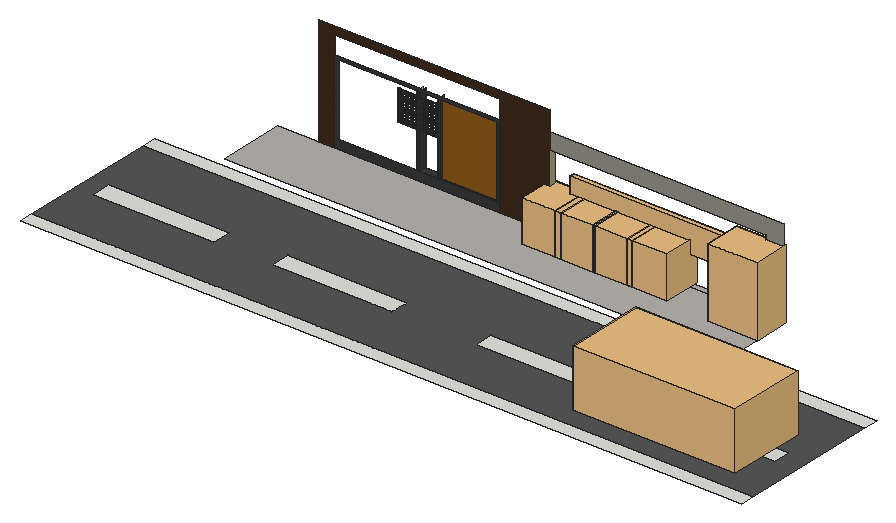
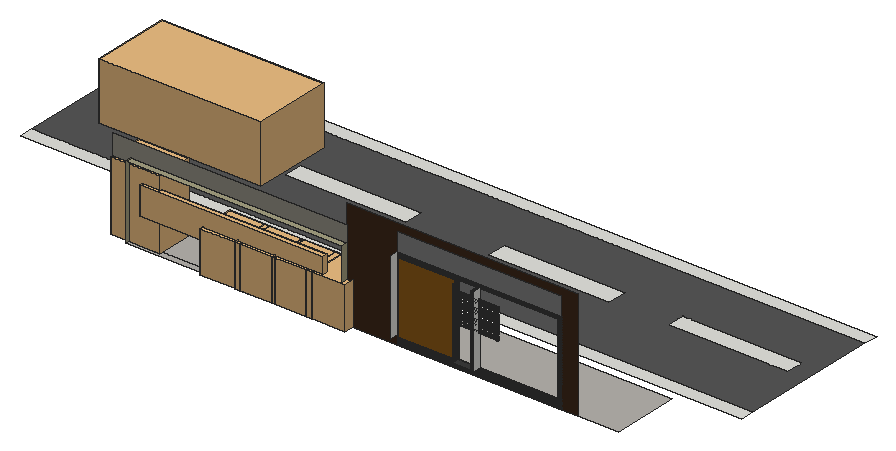
# SketchUp Ruby script. Lengths in inches.
U = 1.inch
M = Sketchup.active_model
def pt(a) = Geom::Point3d.new(a.map { |v| v * U })
def face(e, loops, mat)
  f = e.add_face(loops[0].map { |a| pt(a) })
  loops[1..].each { |l| e.add_face(l.map { |a| pt(a) }).erase! }
  f.material = f.back_material = mat if mat
  f
end
# faces: each face lists its corners as indices into pts; further lists are holes
def faces(e, pts, list, mat = nil) = list.each { |f| face(e, (f[0].is_a?(Array) ? f : [f]).map { |l| l.map { |i| pts[i] } }, mat) }
# xy, xz, yz: faces in a plane at the given z, y or x. An outline is a flat list of corners, or four numbers for a rectangle; further outlines are holes
def ring(l) = l.size == 4 ? [[l[0], l[1]], [l[2], l[1]], [l[2], l[3]], [l[0], l[3]]] : l.each_slice(2).to_a
def flat(e, list, mat, &to3) = list.each { |f| face(e, (f[0].is_a?(Array) ? f : [f]).map { |l| ring(l).map { |u, v| to3.(u, v) } }, mat) }
def xy(e, z, list, mat = nil) = flat(e, list, mat) { |x, y| [x, y, z] }
def xz(e, y, list, mat = nil) = flat(e, list, mat) { |x, z| [x, y, z] }
def yz(e, x, list, mat = nil) = flat(e, list, mat) { |y, z| [x, y, z] }
def lines(e, pts, list) = list.each { |a, b| e.add_line(pt(pts[a]), pt(pts[b])) }
# prism: a flat outline (further loops are holes) pulled along v
def prism(e, loops, v, mat = nil)
  f = face(e, loops, mat); d = Geom::Vector3d.new(v.map { |x| x * U })
  f.pushpull(f.normal.samedirection?(d) ? d.length : -d.length)
end
def box(e, o, s, mat = nil) = prism(e, [[o, [o[0] + s[0], o[1], o[2]], [o[0] + s[0], o[1] + s[1], o[2]], [o[0], o[1] + s[1], o[2]]]], [0, 0, s[2]], mat)
def at(x, y, z, deg = 0) = Geom::Transformation.translation(pt([x, y, z])) * Geom::Transformation.rotation(ORIGIN, Z_AXIS, deg.degrees)
def axes(o, x, y, z) = Geom::Transformation.new([*x, 0, *y, 0, *z, 0, *pt(o).to_a, 1])
def part(name) = M.definitions.add(name)
# library, detail: a bought-in or finely detailed component or shape, given as its bounding box
def library(name, o, s) = part(name).tap { |d| box(d.entities, o, s) }
def detail(e, o, s) = box(e.add_group.entities, o, s)
def put(e, d, t, mat = nil) = e.add_instance(d, t).tap { |i| i.material = mat if mat }
def group(e, t, mat = nil) = e.add_group.tap { |g| g.transformation = t; g.material = mat if mat }.entities
root = M.entities
M.materials.add("[Blinds Weave]").color = [141, 91, 25]
M.materials.add("[Color M06]").color = [86, 86, 86]
M.materials.add("[Color M07]").color = [58, 58, 58]
M.materials.add("[Formica Graystone]1").color = [149, 146, 135]
M.materials.add("[Formica Speckled Grey]").color = [94, 105, 111]
M.materials.add("[Sandstone]").color = [63, 43, 28]
M.materials.add("[Stone Coursed Rough]").color = [165, 160, 130]
M.materials.add("[Tile Travertine 2 inch]").color = [181, 178, 172]
c1 = library("Small+Bush+Planter",[-31.86,3.96,0],[62.63,58.8,106.375])
c2 = library("MVSR Maanus",[1.41,0,0],[199.01,20.125,12])
c3 = library("chau cay",[-24.34,-109.24,0],[56.46,62.58,79.69])
c4 = library("2015 Porsche Macan",[0.14,0.6,0.32],[90.05,184.43,65.58])
xy(root,0,[[0,0,824.125,15.99],[21.05,78.34,158.24,100.09],[225.11,78.34,362.3,100.09],[458.05,78.34,595.24,100.09],[662.36,78.34,799.55,100.09],
  [0,176.43,824.125,192.625]])
xy(root,0,[[[0,15.99,824.125,176.43],[21.05,78.34,158.24,100.09],[225.11,78.34,362.3,100.09],[458.05,78.34,595.24,100.09],[662.36,78.34,799.55,100.09]]],"[Color M06]")
xy(root,0,[[71.32,202.61,649.65,279.21],[381.67,279.21,628.99,285.9]],"[Tile Travertine 2 inch]")
xy(root,10.08,[[229.25,279.21,232.82,288.34]])
xy(root,10.08,[[232.82,279.21,253.76,288.34],[256.89,279.21,321.11,281.7]],"[Color M07]")
xy(root,83.9375,[[381.67,279.21,628.99,285.9]],"[Stone Coursed Rough]")
xz(root,279.21,[[136.3,0,324.42,10.08],[136.3,10.08,140.74,10.08,140.74,91.34,321.11,91.34,321.11,10.08,324.42,10.08,324.42,94.91,136.3,94.91],[229.25,10.08,232.82,91.34],[253.76,10.08,256.89,91.34]],"[Color M07]")
xz(root,279.21,[[628.99,0,649.65,0,649.65,103.14,381.67,103.14,381.67,83.9375,628.99,83.9375]],"[Formica Graystone]1")
xz(root,279.21,[[118.15,0,136.3,0,136.3,116.23,324.42,116.23,324.42,0,381.67,0,381.67,124.77,118.15,124.77]],"[Sandstone]")
xz(root,281.7,[[256.89,10.08,321.11,91.34]],"[Blinds Weave]")
yz(root,229.25,[[279.21,10.08,288.34,91.34]])
yz(root,232.82,[[279.21,10.08,288.34,91.34]],"[Color M07]")
yz(root,253.76,[[[279.21,10.08,288.34,91.34],[283.74,87.76,283.9,87.78,284.05,87.84,284.18,87.94,284.28,88.07,284.34,88.22,284.37,88.38,284.34,88.55,284.28,88.7,284.18,88.83,284.05,88.93,283.9,88.99,283.74,89.01,283.58,88.99,283.43,88.93,283.3,88.83,283.2,88.7,283.14,88.55,283.12,88.38,283.14,88.22,283.2,88.07,283.3,87.94,283.43,87.84,283.58,87.78],[283.74,84.95,283.9,84.97,284.05,85.03,284.18,85.13,284.28,85.26,284.34,85.41,284.37,85.57,284.34,85.73,284.28,85.88,284.18,86.01,284.05,86.11,283.9,86.18,283.74,86.2,283.58,86.18,283.43,86.11,283.3,86.01,283.2,85.88,283.14,85.73,283.12,85.57,283.14,85.41,283.2,85.26,283.3,85.13,283.43,85.03,283.58,84.97],[283.74,82.13,283.9,82.16,284.05,82.22,284.18,82.32,284.28,82.45,284.34,82.6,284.37,82.76,284.34,82.92,284.28,83.07,284.18,83.2,284.05,83.3,283.9,83.36,283.74,83.38,283.58,83.36,283.43,83.3,283.3,83.2,283.2,83.07,283.14,82.92,283.12,82.76,283.14,82.6,283.2,82.45,283.3,82.32,283.43,82.22,283.58,82.16],[283.74,79.32,283.9,79.34,284.05,79.41,284.18,79.5,284.28,79.63,284.34,79.79,284.37,79.95,284.34,80.11,284.28,80.26,284.18,80.39,284.05,80.49,283.9,80.55,283.74,80.57,283.58,80.55,283.43,80.49,283.3,80.39,283.2,80.26,283.14,80.11,283.12,79.95,283.14,79.79,283.2,79.63,283.3,79.5,283.43,79.41,283.58,79.34],[283.74,76.51,283.9,76.53,284.05,76.59,284.18,76.69,284.28,76.82,284.34,76.97,284.37,77.13,284.34,77.3,284.28,77.45,284.18,77.58,284.05,77.68,283.9,77.74,283.74,77.76,283.58,77.74,283.43,77.68,283.3,77.58,283.2,77.45,283.14,77.3,283.12,77.13,283.14,76.97,283.2,76.82,283.3,76.69,283.43,76.59,283.58,76.53],[283.74,73.7,283.9,73.72,284.05,73.78,284.18,73.88,284.28,74.01,284.34,74.16,284.37,74.32,284.34,74.48,284.28,74.63,284.18,74.76,284.05,74.86,283.9,74.93,283.74,74.95,283.58,74.93,283.43,74.86,283.3,74.76,283.2,74.63,283.14,74.48,283.12,74.32,283.14,74.16,283.2,74.01,283.3,73.88,283.43,73.78,283.58,73.72],[283.74,70.88,283.9,70.91,284.05,70.97,284.18,71.07,284.28,71.2,284.34,71.35,284.37,71.51,284.34,71.67,284.28,71.82,284.18,71.95,284.05,72.05,283.9,72.11,283.74,72.13,283.58,72.11,283.43,72.05,283.3,71.95,283.2,71.82,283.14,71.67,283.12,71.51,283.14,71.35,283.2,71.2,283.3,71.07,283.43,70.97,283.58,70.91],[283.74,68.07,283.9,68.09,284.05,68.16,284.18,68.25,284.28,68.38,284.34,68.54,284.37,68.7,284.34,68.86,284.28,69.01,284.18,69.14,284.05,69.24,283.9,69.3,283.74,69.32,283.58,69.3,283.43,69.24,283.3,69.14,283.2,69.01,283.14,68.86,283.12,68.7,283.14,68.54,283.2,68.38,283.3,68.25,283.43,68.16,283.58,68.09],[283.74,65.26,283.9,65.28,284.05,65.34,284.18,65.44,284.28,65.57,284.34,65.72,284.37,65.88,284.34,66.05,284.28,66.2,284.18,66.33,284.05,66.43,283.9,66.49,283.74,66.51,283.58,66.49,283.43,66.43,283.3,66.33,283.2,66.2,283.14,66.05,283.12,65.88,283.14,65.72,283.2,65.57,283.3,65.44,283.43,65.34,283.58,65.28],[283.74,62.45,283.9,62.47,284.05,62.53,284.18,62.63,284.28,62.76,284.34,62.91,284.37,63.07,284.34,63.23,284.28,63.38,284.18,63.51,284.05,63.61,283.9,63.68,283.74,63.7,283.58,63.68,283.43,63.61,283.3,63.51,283.2,63.38,283.14,63.23,283.12,63.07,283.14,62.91,283.2,62.76,283.3,62.63,283.43,62.53,283.58,62.47],[283.74,59.63,283.9,59.66,284.05,59.72,284.18,59.82,284.28,59.95,284.34,60.1,284.37,60.26,284.34,60.42,284.28,60.57,284.18,60.7,284.05,60.8,283.9,60.86,283.74,60.88,283.58,60.86,283.43,60.8,283.3,60.7,283.2,60.57,283.14,60.42,283.12,60.26,283.14,60.1,283.2,59.95,283.3,59.82,283.43,59.72,283.58,59.66],[283.74,56.82,283.9,56.84,284.05,56.91,284.18,57,284.28,57.13,284.34,57.29,284.37,57.45,284.34,57.61,284.28,57.76,284.18,57.89,284.05,57.99,283.9,58.05,283.74,58.07,283.58,58.05,283.43,57.99,283.3,57.89,283.2,57.76,283.14,57.61,283.12,57.45,283.14,57.29,283.2,57.13,283.3,57,283.43,56.91,283.58,56.84],[283.74,54.01,283.9,54.03,284.05,54.09,284.18,54.19,284.28,54.32,284.34,54.47,284.37,54.63,284.34,54.8,284.28,54.95,284.18,55.08,284.05,55.18,283.9,55.24,283.74,55.26,283.58,55.24,283.43,55.18,283.3,55.08,283.2,54.95,283.14,54.8,283.12,54.63,283.14,54.47,283.2,54.32,283.3,54.19,283.43,54.09,283.58,54.03],[283.74,51.2,283.9,51.22,284.05,51.28,284.18,51.38,284.28,51.51,284.34,51.66,284.37,51.82,284.34,51.98,284.28,52.13,284.18,52.26,284.05,52.36,283.9,52.43,283.74,52.45,283.58,52.43,283.43,52.36,283.3,52.26,283.2,52.13,283.14,51.98,283.12,51.82,283.14,51.66,283.2,51.51,283.3,51.38,283.43,51.28,283.58,51.22],[283.74,48.38,283.9,48.41,284.05,48.47,284.18,48.57,284.28,48.7,284.34,48.85,284.37,49.01,284.34,49.17,284.28,49.32,284.18,49.45,284.05,49.55,283.9,49.61,283.74,49.63,283.58,49.61,283.43,49.55,283.3,49.45,283.2,49.32,283.14,49.17,283.12,49.01,283.14,48.85,283.2,48.7,283.3,48.57,283.43,48.47,283.58,48.41],[283.74,45.57,283.9,45.59,284.05,45.66,284.18,45.75,284.28,45.88,284.34,46.04,284.37,46.2,284.34,46.36,284.28,46.51,284.18,46.64,284.05,46.74,283.9,46.8,283.74,46.82,283.58,46.8,283.43,46.74,283.3,46.64,283.2,46.51,283.14,46.36,283.12,46.2,283.14,46.04,283.2,45.88,283.3,45.75,283.43,45.66,283.58,45.59],[283.74,42.26,283.9,42.28,284.05,42.34,284.18,42.44,284.28,42.57,284.34,42.72,284.37,42.88,284.34,43.05,284.28,43.2,284.18,43.33,284.05,43.43,283.9,43.49,283.74,43.51,283.58,43.49,283.43,43.43,283.3,43.33,283.2,43.2,283.14,43.05,283.12,42.88,283.14,42.72,283.2,42.57,283.3,42.44,283.43,42.34,283.58,42.28],[283.74,38.95,283.9,38.97,284.05,39.03,284.18,39.13,284.28,39.26,284.34,39.41,284.37,39.57,284.34,39.73,284.28,39.88,284.18,40.01,284.05,40.11,283.9,40.18,283.74,40.2,283.58,40.18,283.43,40.11,283.3,40.01,283.2,39.88,283.14,39.73,283.12,39.57,283.14,39.41,283.2,39.26,283.3,39.13,283.43,39.03,283.58,38.97],[283.74,35.63,283.9,35.66,284.05,35.72,284.18,35.82,284.28,35.95,284.34,36.1,284.37,36.26,284.34,36.42,284.28,36.57,284.18,36.7,284.05,36.8,283.9,36.86,283.74,36.88,283.58,36.86,283.43,36.8,283.3,36.7,283.2,36.57,283.14,36.42,283.12,36.26,283.14,36.1,283.2,35.95,283.3,35.82,283.43,35.72,283.58,35.66],[283.74,32.32,283.9,32.34,284.05,32.41,284.18,32.5,284.28,32.63,284.34,32.79,284.37,32.95,284.34,33.11,284.28,33.26,284.18,33.39,284.05,33.49,283.9,33.55,283.74,33.57,283.58,33.55,283.43,33.49,283.3,33.39,283.2,33.26,283.14,33.11,283.12,32.95,283.14,32.79,283.2,32.63,283.3,32.5,283.43,32.41,283.58,32.34],[283.74,29.01,283.9,29.03,284.05,29.09,284.18,29.19,284.28,29.32,284.34,29.47,284.37,29.63,284.34,29.8,284.28,29.95,284.18,30.08,284.05,30.18,283.9,30.24,283.74,30.26,283.58,30.24,283.43,30.18,283.3,30.08,283.2,29.95,283.14,29.8,283.12,29.63,283.14,29.47,283.2,29.32,283.3,29.19,283.43,29.09,283.58,29.03],[283.74,25.7,283.9,25.72,284.05,25.78,284.18,25.88,284.28,26.01,284.34,26.16,284.37,26.32,284.34,26.48,284.28,26.63,284.18,26.76,284.05,26.86,283.9,26.93,283.74,26.95,283.58,26.93,283.43,26.86,283.3,26.76,283.2,26.63,283.14,26.48,283.12,26.32,283.14,26.16,283.2,26.01,283.3,25.88,283.43,25.78,283.58,25.72],[283.74,12.45,283.9,12.47,284.05,12.53,284.18,12.63,284.28,12.76,284.34,12.91,284.37,13.07,284.34,13.23,284.28,13.38,284.18,13.51,284.05,13.61,283.9,13.68,283.74,13.7,283.58,13.68,283.43,13.61,283.3,13.51,283.2,13.38,283.14,13.23,283.12,13.07,283.14,12.91,283.2,12.76,283.3,12.63,283.43,12.53,283.58,12.47],[283.74,15.76,283.9,15.78,284.05,15.84,284.18,15.94,284.28,16.07,284.34,16.22,284.37,16.38,284.34,16.55,284.28,16.7,284.18,16.83,284.05,16.93,283.9,16.99,283.74,17.01,283.58,16.99,283.43,16.93,283.3,16.83,283.2,16.7,283.14,16.55,283.12,16.38,283.14,16.22,283.2,16.07,283.3,15.94,283.43,15.84,283.58,15.78],[283.74,22.38,283.9,22.41,284.05,22.47,284.18,22.57,284.28,22.7,284.34,22.85,284.37,23.01,284.34,23.17,284.28,23.32,284.18,23.45,284.05,23.55,283.9,23.61,283.74,23.63,283.58,23.61,283.43,23.55,283.3,23.45,283.2,23.32,283.14,23.17,283.12,23.01,283.14,22.85,283.2,22.7,283.3,22.57,283.43,22.47,283.58,22.41],[283.74,19.07,283.9,19.09,284.05,19.16,284.18,19.25,284.28,19.38,284.34,19.54,284.37,19.7,284.34,19.86,284.28,20.01,284.18,20.14,284.05,20.24,283.9,20.3,283.74,20.32,283.58,20.3,283.43,20.24,283.3,20.14,283.2,20.01,283.14,19.86,283.12,19.7,283.14,19.54,283.2,19.38,283.3,19.25,283.43,19.16,283.58,19.09]]],"[Color M07]")
yz(root,256.89,[[279.21,10.08,281.7,91.34]],"[Color M07]")
yz(root,321.11,[[279.21,10.08,281.7,91.34]],"[Color M07]")
yz(root,324.42,[[279.21,10.08,288.34,94.91]])
yz(root,381.67,[[279.21,0,285.9,10.08],[279.21,10.08,285.9,83.9375]],"[Stone Coursed Rough]")
yz(root,628.99,[[279.21,0,285.9,83.9375]],"[Stone Coursed Rough]")
p = [[204.61,283.43,48.47],[204.61,283.58,48.41],[253.76,283.58,48.41],[253.76,283.43,48.47],[204.61,283.74,48.38],[253.76,283.74,48.38],
  [204.61,283.3,48.57],[253.76,283.3,48.57],[204.61,283.2,48.7],[253.76,283.2,48.7],[204.61,283.14,48.85],[253.76,283.14,48.85],
  [204.61,283.2,49.32],[204.61,283.14,49.17],[253.76,283.14,49.17],[253.76,283.2,49.32],[204.61,283.3,49.45],[253.76,283.3,49.45],
  [204.61,283.43,49.55],[253.76,283.43,49.55],[204.61,283.58,49.61],[253.76,283.58,49.61],[204.61,283.74,49.63],[253.76,283.74,49.63],
  [204.61,283.43,51.28],[204.61,283.58,51.22],[253.76,283.58,51.22],[253.76,283.43,51.28],[204.61,283.74,51.2],[253.76,283.74,51.2],
  [204.61,283.3,51.38],[253.76,283.3,51.38],[204.61,283.2,51.51],[253.76,283.2,51.51],[204.61,283.14,51.66],[253.76,283.14,51.66],
  [204.61,283.12,51.82],[253.76,283.12,51.82],[204.61,283.14,51.98],[253.76,283.14,51.98],[204.61,283.2,52.13],[253.76,283.2,52.13],
  [204.61,283.3,52.26],[253.76,283.3,52.26],[204.61,283.43,52.36],[253.76,283.43,52.36],[204.61,283.58,52.43],[253.76,283.58,52.43],
  [204.61,283.74,52.45],[253.76,283.74,52.45],[204.61,283.43,54.09],[204.61,283.58,54.03],[253.76,283.58,54.03],[253.76,283.43,54.09],
  [204.61,283.74,54.01],[253.76,283.74,54.01],[204.61,283.3,54.19],[253.76,283.3,54.19],[204.61,283.2,54.32],[253.76,283.2,54.32],
  [204.61,283.14,54.47],[253.76,283.14,54.47],[204.61,283.12,54.63],[253.76,283.12,54.63],[204.61,283.14,54.8],[253.76,283.14,54.8],
  [204.61,283.2,54.95],[253.76,283.2,54.95],[204.61,283.3,55.08],[253.76,283.3,55.08],[204.61,283.43,55.18],[253.76,283.43,55.18],
  [204.61,283.58,55.24],[253.76,283.58,55.24],[204.61,283.74,55.26],[253.76,283.74,55.26],[204.61,283.43,56.91],[204.61,283.58,56.84],
  [253.76,283.58,56.84],[253.76,283.43,56.91],[204.61,283.74,56.82],[253.76,283.74,56.82],[204.61,283.3,57],[253.76,283.3,57],
  [204.61,283.2,57.13],[253.76,283.2,57.13],[204.61,283.14,57.29],[253.76,283.14,57.29],[204.61,283.12,57.45],[253.76,283.12,57.45],
  [204.61,283.14,57.61],[253.76,283.14,57.61],[204.61,283.2,57.76],[253.76,283.2,57.76],[204.61,283.3,57.89],[253.76,283.3,57.89],
  [204.61,283.43,57.99],[253.76,283.43,57.99],[204.61,283.58,58.05],[253.76,283.58,58.05],[204.61,283.74,58.07],[253.76,283.74,58.07],
  [204.61,283.58,59.66],[204.61,283.74,59.63],[253.76,283.74,59.63],[253.76,283.58,59.66],[204.61,283.3,59.82],[204.61,283.43,59.72],
  [253.76,283.43,59.72],[253.76,283.3,59.82],[204.61,283.2,59.95],[253.76,283.2,59.95],[204.61,283.14,60.1],[253.76,283.14,60.1],
  [204.61,283.12,60.26],[253.76,283.12,60.26],[204.61,283.14,60.42],[253.76,283.14,60.42],[204.61,283.2,60.57],[253.76,283.2,60.57],
  [204.61,283.3,60.7],[253.76,283.3,60.7],[204.61,283.43,60.8],[253.76,283.43,60.8],[204.61,283.58,60.86],[253.76,283.58,60.86],
  [204.61,283.74,60.88],[253.76,283.74,60.88],[204.61,283.58,62.47],[204.61,283.74,62.45],[253.76,283.74,62.45],[253.76,283.58,62.47],
  [204.61,283.3,62.63],[204.61,283.43,62.53],[253.76,283.43,62.53],[253.76,283.3,62.63],[204.61,283.2,62.76],[253.76,283.2,62.76],
  [204.61,283.14,62.91],[253.76,283.14,62.91],[204.61,283.12,63.07],[253.76,283.12,63.07],[204.61,283.14,63.23],[253.76,283.14,63.23],
  [204.61,283.2,63.38],[253.76,283.2,63.38],[204.61,283.3,63.51],[253.76,283.3,63.51],[204.61,283.43,63.61],[253.76,283.43,63.61],
  [204.61,283.58,63.68],[253.76,283.58,63.68],[204.61,283.74,63.7],[253.76,283.74,63.7],[204.61,283.3,65.44],[204.61,283.43,65.34],
  [253.76,283.43,65.34],[253.76,283.3,65.44],[204.61,283.58,65.28],[253.76,283.58,65.28],[204.61,283.74,65.26],[253.76,283.74,65.26],
  [204.61,283.2,65.57],[253.76,283.2,65.57],[204.61,283.14,65.72],[253.76,283.14,65.72],[204.61,283.12,65.88],[253.76,283.12,65.88],
  [204.61,283.14,66.05],[253.76,283.14,66.05],[204.61,283.2,66.2],[253.76,283.2,66.2],[204.61,283.3,66.33],[253.76,283.3,66.33],
  [204.61,283.43,66.43],[253.76,283.43,66.43],[204.61,283.58,66.49],[253.76,283.58,66.49],[204.61,283.74,66.51],[253.76,283.74,66.51],
  [204.61,283.43,68.16],[204.61,283.58,68.09],[253.76,283.58,68.09],[253.76,283.43,68.16],[204.61,283.74,68.07],[253.76,283.74,68.07],
  [204.61,283.3,68.25],[253.76,283.3,68.25],[204.61,283.2,68.38],[253.76,283.2,68.38],[204.61,283.14,68.54],[253.76,283.14,68.54],
  [204.61,283.12,68.7],[253.76,283.12,68.7],[204.61,283.14,68.86],[253.76,283.14,68.86],[204.61,283.2,69.01],[253.76,283.2,69.01],
  [204.61,283.3,69.14],[253.76,283.3,69.14],[204.61,283.43,69.24],[253.76,283.43,69.24],[204.61,283.58,69.3],[253.76,283.58,69.3],
  [204.61,283.74,69.32],[253.76,283.74,69.32],[204.61,283.43,70.97],[204.61,283.58,70.91],[253.76,283.58,70.91],[253.76,283.43,70.97],
  [204.61,283.74,70.88],[253.76,283.74,70.88],[204.61,283.3,71.07],[253.76,283.3,71.07],[204.61,283.2,71.2],[253.76,283.2,71.2],
  [204.61,283.14,71.35],[253.76,283.14,71.35],[204.61,283.12,71.51],[253.76,283.12,71.51],[204.61,283.14,71.67],[253.76,283.14,71.67],
  [204.61,283.2,71.82],[253.76,283.2,71.82],[204.61,283.3,71.95],[253.76,283.3,71.95],[204.61,283.43,72.05],[253.76,283.43,72.05],
  [204.61,283.58,72.11],[253.76,283.58,72.11],[204.61,283.74,72.13],[253.76,283.74,72.13],[204.61,283.43,73.78],[204.61,283.58,73.72],
  [253.76,283.58,73.72],[253.76,283.43,73.78],[204.61,283.74,73.7],[253.76,283.74,73.7],[204.61,283.3,73.88],[253.76,283.3,73.88],
  [204.61,283.2,74.01],[253.76,283.2,74.01],[204.61,283.14,74.16],[253.76,283.14,74.16],[204.61,283.12,74.32],[253.76,283.12,74.32],
  [204.61,283.14,74.48],[253.76,283.14,74.48],[204.61,283.2,74.63],[253.76,283.2,74.63],[204.61,283.3,74.76],[253.76,283.3,74.76],
  [204.61,283.43,74.86],[253.76,283.43,74.86],[204.61,283.58,74.93],[253.76,283.58,74.93],[204.61,283.74,74.95],[253.76,283.74,74.95],
  [204.61,283.43,76.59],[204.61,283.58,76.53],[253.76,283.58,76.53],[253.76,283.43,76.59],[204.61,283.74,76.51],[253.76,283.74,76.51],
  [204.61,283.3,76.69],[253.76,283.3,76.69],[204.61,283.2,76.82],[253.76,283.2,76.82],[204.61,283.14,76.97],[253.76,283.14,76.97],
  [204.61,283.12,77.13],[253.76,283.12,77.13],[204.61,283.14,77.3],[253.76,283.14,77.3],[204.61,283.2,77.45],[253.76,283.2,77.45],
  [204.61,283.3,77.58],[253.76,283.3,77.58],[204.61,283.43,77.68],[253.76,283.43,77.68],[204.61,283.58,77.74],[253.76,283.58,77.74],
  [204.61,283.74,77.76],[253.76,283.74,77.76],[204.61,283.43,79.41],[204.61,283.58,79.34],[253.76,283.58,79.34],[253.76,283.43,79.41],
  [204.61,283.74,79.32],[253.76,283.74,79.32],[204.61,283.3,79.5],[253.76,283.3,79.5],[204.61,283.2,79.63],[253.76,283.2,79.63],
  [204.61,283.14,79.79],[253.76,283.14,79.79],[204.61,283.12,79.95],[253.76,283.12,79.95],[204.61,283.14,80.11],[253.76,283.14,80.11],
  [204.61,283.2,80.26],[253.76,283.2,80.26],[204.61,283.3,80.39],[253.76,283.3,80.39],[204.61,283.43,80.49],[253.76,283.43,80.49],
  [204.61,283.58,80.55],[253.76,283.58,80.55],[204.61,283.74,80.57],[253.76,283.74,80.57],[204.61,283.58,82.16],[204.61,283.74,82.13],
  [253.76,283.74,82.13],[253.76,283.58,82.16],[204.61,283.3,82.32],[204.61,283.43,82.22],[253.76,283.43,82.22],[253.76,283.3,82.32],
  [204.61,283.2,82.45],[253.76,283.2,82.45],[204.61,283.14,82.6],[253.76,283.14,82.6],[204.61,283.12,82.76],[253.76,283.12,82.76],
  [204.61,283.14,82.92],[253.76,283.14,82.92],[204.61,283.2,83.07],[253.76,283.2,83.07],[204.61,283.3,83.2],[253.76,283.3,83.2],
  [204.61,283.43,83.3],[253.76,283.43,83.3],[204.61,283.58,83.36],[253.76,283.58,83.36],[204.61,283.74,83.38],[253.76,283.74,83.38]]
faces(root,p,[[0,1,2,3],[1,4,5,2],[6,0,3,7],[8,6,7,9],[10,8,9,11],[12,13,14,15],[16,12,15,17],[18,16,17,19],
  [20,18,19,21],[22,20,21,23],[24,25,26,27],[25,28,29,26],[30,24,27,31],[32,30,31,33],[34,32,33,35],[36,34,35,37],
  [38,36,37,39],[40,38,39,41],[42,40,41,43],[44,42,43,45],[46,44,45,47],[48,46,47,49],[50,51,52,53],[51,54,55,52],
  [56,50,53,57],[58,56,57,59],[60,58,59,61],[62,60,61,63],[64,62,63,65],[66,64,65,67],[68,66,67,69],[70,68,69,71],
  [72,70,71,73],[74,72,73,75],[76,77,78,79],[77,80,81,78],[82,76,79,83],[84,82,83,85],[86,84,85,87],[88,86,87,89],
  [90,88,89,91],[92,90,91,93],[94,92,93,95],[96,94,95,97],[98,96,97,99],[100,98,99,101],[102,103,104,105],[106,107,108,109],
  [107,102,105,108],[110,106,109,111],[112,110,111,113],[114,112,113,115],[116,114,115,117],[118,116,117,119],[120,118,119,121],[122,120,121,123],
  [124,122,123,125],[126,124,125,127],[128,129,130,131],[132,133,134,135],[133,128,131,134],[136,132,135,137],[138,136,137,139],[140,138,139,141],
  [142,140,141,143],[144,142,143,145],[146,144,145,147],[148,146,147,149],[150,148,149,151],[152,150,151,153],[154,155,156,157],[155,158,159,156],
  [158,160,161,159],[162,154,157,163],[164,162,163,165],[166,164,165,167],[168,166,167,169],[170,168,169,171],[172,170,171,173],[174,172,173,175],
  [176,174,175,177],[178,176,177,179],[180,181,182,183],[181,184,185,182],[186,180,183,187],[188,186,187,189],[190,188,189,191],[192,190,191,193],
  [194,192,193,195],[196,194,195,197],[198,196,197,199],[200,198,199,201],[202,200,201,203],[204,202,203,205],[206,207,208,209],[207,210,211,208],
  [212,206,209,213],[214,212,213,215],[216,214,215,217],[218,216,217,219],[220,218,219,221],[222,220,221,223],[224,222,223,225],[226,224,225,227],
  [228,226,227,229],[230,228,229,231],[232,233,234,235],[233,236,237,234],[238,232,235,239],[240,238,239,241],[242,240,241,243],[244,242,243,245],
  [246,244,245,247],[248,246,247,249],[250,248,249,251],[252,250,251,253],[254,252,253,255],[256,254,255,257],[258,259,260,261],[259,262,263,260],
  [264,258,261,265],[266,264,265,267],[268,266,267,269],[270,268,269,271],[272,270,271,273],[274,272,273,275],[276,274,275,277],[278,276,277,279],
  [280,278,279,281],[282,280,281,283],[284,285,286,287],[285,288,289,286],[290,284,287,291],[292,290,291,293],[294,292,293,295],[296,294,295,297],
  [298,296,297,299],[300,298,299,301],[302,300,301,303],[304,302,303,305],[306,304,305,307],[308,306,307,309],[310,311,312,313],[314,315,316,317],
  [315,310,313,316],[318,314,317,319],[320,318,319,321],[322,320,321,323],[324,322,323,325],[326,324,325,327],[328,326,327,329],[330,328,329,331],
  [332,330,331,333],[334,332,333,335]],"[Formica Speckled Grey]")
put(root,c1,axes([398.34,244.19,0],[0.72,0,0],[0,0.72,0],[0,0,0.4464]))
put(root,c1,axes([436.59,244.19,0],[0.72,0,0],[0,0.72,0],[0,0,0.4464]))
put(root,c1,axes([479.02,244.19,0],[0.72,0,0],[0,0.72,0],[0,0,0.4464]))
put(root,c2,axes([402.37,285.9,33.63],[1.05,0,0],[0,0,1.56],[0,-0.5,0]),"[Color M07]")
put(root,c1,axes([518.96,244.19,0],[0.72,0,0],[0,0.72,0],[0,0,0.4464]))
put(root,c3,axes([617.53,311.92,0],[1,0,0],[0,0.65,0],[0,0,1]))
put(root,c4,at(599.63,129.69,-0.32,-90))
